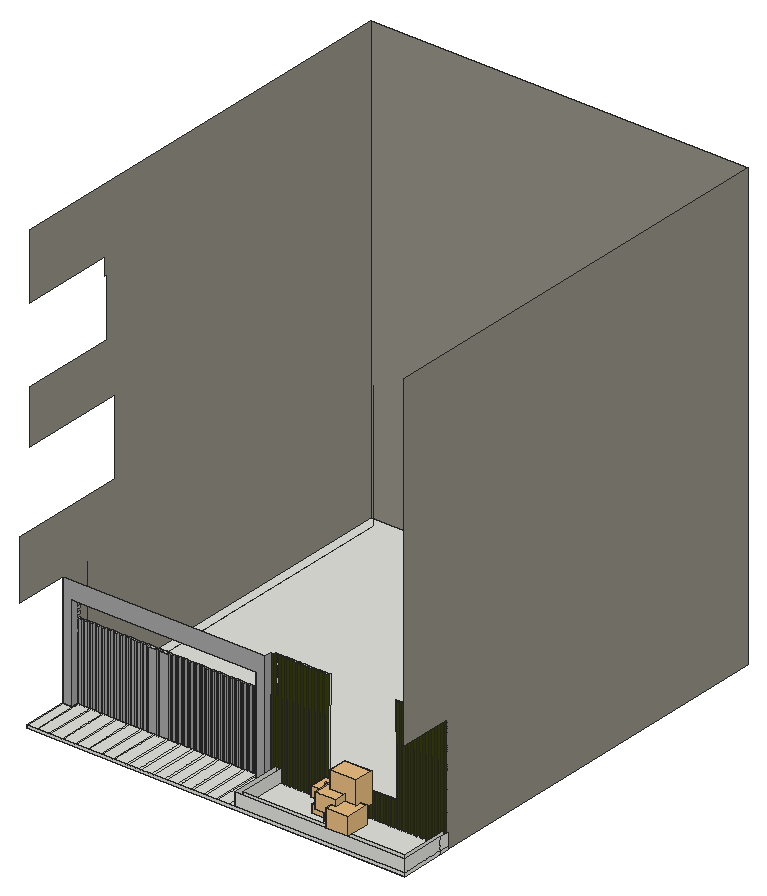
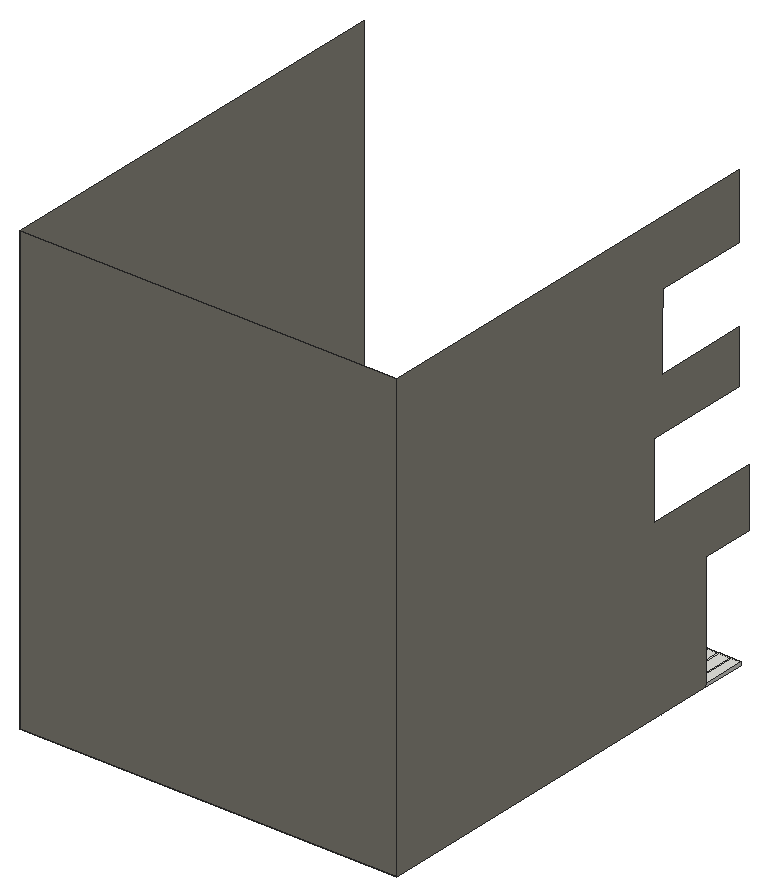
# SketchUp Ruby script. Lengths in inches.
U = 1.inch
M = Sketchup.active_model
def pt(a) = Geom::Point3d.new(a.map { |v| v * U })
def face(e, loops, mat)
  f = e.add_face(loops[0].map { |a| pt(a) })
  loops[1..].each { |l| e.add_face(l.map { |a| pt(a) }).erase! }
  f.material = f.back_material = mat if mat
  f
end
# faces: each face lists its corners as indices into pts; further lists are holes
def faces(e, pts, list, mat = nil) = list.each { |f| face(e, (f[0].is_a?(Array) ? f : [f]).map { |l| l.map { |i| pts[i] } }, mat) }
# xy, xz, yz: faces in a plane at the given z, y or x. An outline is a flat list of corners, or four numbers for a rectangle; further outlines are holes
def ring(l) = l.size == 4 ? [[l[0], l[1]], [l[2], l[1]], [l[2], l[3]], [l[0], l[3]]] : l.each_slice(2).to_a
def flat(e, list, mat, &to3) = list.each { |f| face(e, (f[0].is_a?(Array) ? f : [f]).map { |l| ring(l).map { |u, v| to3.(u, v) } }, mat) }
def xy(e, z, list, mat = nil) = flat(e, list, mat) { |x, y| [x, y, z] }
def xz(e, y, list, mat = nil) = flat(e, list, mat) { |x, z| [x, y, z] }
def yz(e, x, list, mat = nil) = flat(e, list, mat) { |y, z| [x, y, z] }
def lines(e, pts, list) = list.each { |a, b| e.add_line(pt(pts[a]), pt(pts[b])) }
# prism: a flat outline (further loops are holes) pulled along v
def prism(e, loops, v, mat = nil)
  f = face(e, loops, mat); d = Geom::Vector3d.new(v.map { |x| x * U })
  f.pushpull(f.normal.samedirection?(d) ? d.length : -d.length)
end
def box(e, o, s, mat = nil) = prism(e, [[o, [o[0] + s[0], o[1], o[2]], [o[0] + s[0], o[1] + s[1], o[2]], [o[0], o[1] + s[1], o[2]]]], [0, 0, s[2]], mat)
def at(x, y, z, deg = 0) = Geom::Transformation.translation(pt([x, y, z])) * Geom::Transformation.rotation(ORIGIN, Z_AXIS, deg.degrees)
def axes(o, x, y, z) = Geom::Transformation.new([*x, 0, *y, 0, *z, 0, *pt(o).to_a, 1])
def part(name) = M.definitions.add(name)
# library, detail: a bought-in or finely detailed component or shape, given as its bounding box
def library(name, o, s) = part(name).tap { |d| box(d.entities, o, s) }
def detail(e, o, s) = box(e.add_group.entities, o, s)
def put(e, d, t, mat = nil) = e.add_instance(d, t).tap { |i| i.material = mat if mat }
def group(e, t, mat = nil) = e.add_group.tap { |g| g.transformation = t; g.material = mat if mat }.entities
root = M.entities
M.materials.add("Material__1").color = [95, 70, 46]
M.materials.add("Material__2").color = [150, 168, 104]
M.materials.add("Material__3").color = [234, 233, 231]
M.materials.add("Material__4").color = [36, 36, 36]
M.materials.add("Material__5").color = [151, 172, 33]
M.materials.add("Material__6").color = [79, 108, 5]
M.materials.add("[0043_SaddleBrown]1").color = [58, 63, 9]
M.materials.add("[0132_LightGray]").color = [169, 169, 169]
M.materials.add("[Formica Graystone]").color = [149, 146, 135]
M.materials.add("[Polished Concrete Old]").color = [168, 168, 168]
M.materials.add("wire_1").color = [140, 184, 58]
M.materials.add("wire_2").color = [244, 244, 244]
M.materials.add("wire_4").color = [86, 225, 198]
M.materials.add("wire_5").color = [232, 232, 232]
c1 = library("Group\#1",[-915.9375,-34.5,735.6],[41.04,40.85,6.81])
c2 = library("Group\#2",[-991.92,-34.05,729.49],[10.64,7.28,57.53])
c3 = library("Group\#3",[-1022.2,-71.69,736.68],[86.94,78.77,45.64])
c4 = library("Group\#4",[-877.77,-100.41,669.81],[37.9,37.9,42.75])
c5 = library("Group\#5",[-957.79,-83.08,701.98],[44.29,44.29,27.78])
c6 = library("Group\#6",[-1023.9,-65.47,669.625],[67.53,67.55,39.17])
c7 = library("Group\#7",[-997.48,-49.45,708.79],[29.81,29.81,30.61])
c8 = library("Group\#8",[-956738.95,-82059.81,669752.625],[42194.58,42232.57,49521.48])
c9 = library("Group\#9",[-917.52,-36.6875,711.84],[44.99,44.98,28.22])
c10 = library("Group\#10",[-916244.63,-35413.97,669800.48],[42442.38,42642.99,59706.29])
c11 = library("Group\#11",[-955.48,-54.29,730.4],[118.63,83.7,130.4])
c12 = library("Group\#12",[-899.97,-18.72,732.17],[8.78,8.27,28.64])
c13 = library("Group\#13",[-906.16,-138.28,686.8],[98.25,106.18,75.79])
c14 = library("Group\#14",[-978.71,-103.24,719.12],[90.2,76.4,68.29])
c15 = library("Group\#15",[-955.98,-81.17,725.57],[41.03,40.85,6.81])
c16 = library("Group\#16",[-996.8,-48.73,736.67],[28.51,28.38,4.73])
c17 = library("Group\#17",[-876.58,-99.29,706.19],[35.74,35.58,5.93])
c18 = library("Group\#18",[-912.1,-32.49,735.82],[33.14,36.63,9.55])
c19 = library("Group\#19",[-994.36,-46.95,735.88],[24.38,25.9,6.88])
c20 = part("PLANT-30")
p = [[0,0,0],[1,0,0],[1,1,0]]
lines(c20.entities,p,[[0,1],[1,2],[2,0]])
put(c20.entities,c1,at(895.63,-7.06,-669.82),"Material__1")
put(c20.entities,c2,at(895.63,-7.06,-669.82),"wire_1")
put(c20.entities,c3,at(895.63,-7.06,-669.82),"Material__2")
put(c20.entities,c4,at(895.63,-7.06,-669.82),"wire_2")
put(c20.entities,c5,at(895.63,-7.06,-669.82),"wire_2")
put(c20.entities,c6,at(895.63,-7.06,-669.82),"Material__3")
put(c20.entities,c7,at(895.63,-7.06,-669.82),"wire_2")
put(c20.entities,c8,axes([895.63,-7.06,-669.82],[0.001,0,0],[0,0.001,0],[0,0,0.001]),"Material__4")
put(c20.entities,c9,at(895.63,-7.06,-669.82),"wire_2")
put(c20.entities,c10,axes([895.63,-7.06,-669.82],[0.001,0,0],[0,0.001,0],[0,0,0.001]),"Material__4")
put(c20.entities,c11,at(895.63,-7.06,-669.82),"Material__5")
put(c20.entities,c12,at(895.63,-7.06,-669.82),"wire_4")
put(c20.entities,c13,at(895.63,-7.06,-669.82),"Material__6")
put(c20.entities,c14,at(895.63,-7.06,-669.82),"Material__4")
put(c20.entities,c15,at(895.63,-7.06,-669.82),"Material__1")
put(c20.entities,c16,at(895.63,-7.06,-669.82),"Material__1")
put(c20.entities,c17,at(895.63,-7.06,-669.82),"Material__1")
put(c20.entities,c18,at(895.63,-7.06,-669.82),"wire_5")
put(c20.entities,c19,at(895.63,-7.06,-669.82),"wire_5")
xy(root,0,[[0,17.5625,361.1875,60],[0,60,0,429,360,429,360,69,196.36,69,196.36,68.9375,193.125,68.9375,193.125,69,8.86,69,8.86,60],[8.86,60,184.43,66],[184.43,60,193.125,69],[193.125,60,193.125,67,196.36,67,196.36,68.9375,198.375,68.9375,198.375,67,201.61,67,201.61,68.9375,203.625,68.9375,203.625,67,206.86,67,206.86,68.9375,208.875,68.9375,208.875,67,212.11,67,212.11,68.9375,214.125,68.9375,214.125,67,217.36,67,217.36,68.9375,219.375,68.9375,219.375,67,222.61,67,222.61,68.9375,224.625,68.9375,224.625,67,227.86,67,227.86,68.9375,229.875,68.9375,229.875,67,233.11,67,233.11,68.9375,235.125,68.9375,235.125,67,238.36,67,238.36,68.9375,240.375,68.9375,240.375,67,243.61,67,243.61,68.9375,245.625,68.9375,245.625,67,248.86,67,248.86,68.9375,250.875,68.9375,250.875,67,254.11,67,254.11,68.9375,256.125,68.9375,256.125,67,259.36,67,259.36,68.9375,261.375,68.9375,261.375,67,264.61,67,264.61,68.9375,266.625,68.9375,266.625,67,269.86,67,269.86,68.9375,271.875,68.9375,271.875,67,275.11,67,275.11,68.9375,277.125,68.9375,277.125,67,280.36,67,280.36,68.9375,282.375,68.9375,282.375,67,285.61,67,285.61,68.9375,287.625,68.9375,287.625,67,290.86,67,290.86,68.9375,292.875,68.9375,292.875,67,296.11,67,296.11,68.9375,298.125,68.9375,298.125,67,301.36,67,301.36,68.9375,303.375,68.9375,303.375,67,306.61,67,306.61,68.9375,308.625,68.9375,308.625,67,311.86,67,311.86,68.9375,313.875,68.9375,313.875,67,317.11,67,317.11,68.9375,319.125,68.9375,319.125,67,322.36,67,322.36,68.9375,324.375,68.9375,324.375,67,327.61,67,327.61,68.9375,330.125,68.9375,330.125,67,333.36,67,333.36,68.9375,335.875,68.9375,335.875,67,339.11,67,339.11,68.9375,341.625,68.9375,341.625,67,344.86,67,344.86,68.9375,347.375,68.9375,347.375,67,350.61,67,350.61,68.9375,353.125,68.9375,353.125,67,356.36,67,356.36,68.9375,358.875,68.9375,358.875,67,360,67,360,68.9375,361.1875,68.9375,361.1875,60],
  [76.57,66,85.45,69],[87.63,66,96.52,69],[8.86,67,12.35,69],[14.55,67,18.04,69],[20.24,67,23.72,69],
  [25.93,67,29.41,69],[31.61,67,35.1,69],[37.3,67,40.79,69],[42.99,67,46.47,69],[48.68,67,52.16,69],
  [54.36,67,57.85,69],[60.05,67,63.54,69],[65.74,67,69.22,69],[71.43,67,74.91,69],[97.66,67,99.86,69],
  [103.35,67,105.55,69],[109.04,67,111.24,69],[114.72,67,116.93,69],[120.41,67,122.61,69],[126.1,67,128.3,69],
  [131.79,67,133.99,69],[137.47,67,139.68,69],[143.16,67,145.36,69],[148.85,67,151.05,69],[154.54,67,156.74,69],
  [160.22,67,162.43,69],[165.91,67,168.11,69],[171.6,67,173.8,69],[177.29,67,179.49,69],[182.97,67,184.43,69],
  [193.125,67,196.36,68.9375],[198.375,67,201.61,68.9375],[203.625,67,206.86,68.9375],[208.875,67,212.11,68.9375],[214.125,67,217.36,68.9375],
  [219.375,67,222.61,68.9375],[224.625,67,227.86,68.9375],[229.875,67,233.11,68.9375],[235.125,67,238.36,68.9375],[240.375,67,243.61,68.9375],
  [245.625,67,248.86,68.9375],[250.875,67,254.11,68.9375],[256.125,67,259.36,68.9375],[261.375,67,264.61,68.9375],[266.625,67,269.86,68.9375],
  [271.875,67,275.11,68.9375],[277.125,67,280.36,68.9375],[282.375,67,285.61,68.9375],[287.625,67,290.86,68.9375],[292.875,67,296.11,68.9375],
  [298.125,67,301.36,68.9375],[303.375,67,306.61,68.9375],[308.625,67,311.86,68.9375],[313.875,67,317.11,68.9375],[319.125,67,322.36,68.9375],
  [324.375,67,327.61,68.9375],[330.125,67,333.36,68.9375],[335.875,67,339.11,68.9375],[341.625,67,344.86,68.9375],[347.375,67,350.61,68.9375],
  [353.125,67,356.36,68.9375],[358.875,67,360,68.9375],[198.375,68.9375,201.61,69],[203.625,68.9375,206.86,69],[208.875,68.9375,212.11,69],
  [214.125,68.9375,217.36,69],[219.375,68.9375,222.61,69],[224.625,68.9375,227.86,69],[229.875,68.9375,233.11,69],[235.125,68.9375,238.36,69],
  [240.375,68.9375,243.61,69],[245.625,68.9375,248.86,69],[250.875,68.9375,254.11,69],[256.125,68.9375,259.36,69],[261.375,68.9375,264.61,69],
  [266.625,68.9375,269.86,69],[271.875,68.9375,275.11,69],[277.125,68.9375,280.36,69],[282.375,68.9375,285.61,69],[287.625,68.9375,290.86,69],
  [292.875,68.9375,296.11,69],[298.125,68.9375,301.36,69],[303.375,68.9375,306.61,69],[308.625,68.9375,311.86,69],[313.875,68.9375,317.11,69],
  [319.125,68.9375,322.36,69],[324.375,68.9375,327.61,69],[330.125,68.9375,333.36,69],[335.875,68.9375,339.11,69],[341.625,68.9375,344.86,69],
  [347.375,68.9375,350.61,69],[353.125,68.9375,356.36,69],[358.875,68.9375,360,69]])
xy(root,3,[[0,17.5625,9.02,60],[9.02,17.5625,10.37,17.5625,10.37,66,8.86,66,8.86,60,9.02,60],[10.37,17.5625,20.81,66],[20.81,17.5625,22.68,66],[22.68,17.5625,33.12,66],
  [33.12,17.5625,35,66],[35,17.5625,45.43,66],[45.43,17.5625,47.31,66],[47.31,17.5625,57.75,66],[57.75,17.5625,59.62,66],
  [59.62,17.5625,70.06,66],[70.06,17.5625,71.93,66],[71.93,17.5625,82.37,66],[82.37,17.5625,84.25,66],[84.25,17.5625,94.68,66],
  [94.68,17.5625,96.56,66],[96.56,17.5625,107,66],[107,17.5625,108.87,66],[108.87,17.5625,119.31,66],[119.31,17.5625,121.18,66],
  [121.18,17.5625,131.62,66],[131.62,17.5625,133.5,66],[133.5,17.5625,143.93,66],[143.93,17.5625,145.81,66],[145.81,17.5625,156.25,66],
  [156.25,17.5625,158.12,66],[158.12,17.5625,168.56,66],[168.56,17.5625,170.43,66],[170.43,17.5625,180.87,66],[180.87,17.5625,182.75,66],
  [182.75,17.5625,193.18,17.5625,193.18,66,193.125,66,193.125,60,184.43,60,184.43,66,182.75,66],[193.18,17.5625,198.375,17.5625,198.375,67,202.875,67,202.875,22.19,357.51,22.19,357.51,68.9375,193.125,68.9375,193.125,66,193.18,66],[198.375,17.5625,198.375,67,202.875,67,202.875,22.19,357.51,22.19,357.51,68.9375,361.1875,68.9375,361.1875,17.5625],[184.43,60,193.125,66]])
xz(root,17.5625,[[0,0,361.1875,3],[198.375,3,361.1875,15]])
xz(root,22.19,[[202.875,3,357.51,15]])
xz(root,60,[[0,0,8.86,3],[184.43,0,193.125,3]])
xz(root,60,[[0,3,8.86,3,8.86,94.26,184.43,94.26,184.43,3,193.125,3,193.125,111.13,0,111.13]],"[Polished Concrete Old]")
xz(root,66,[[8.86,0,76.57,3],[76.57,0,85.45,3],[85.45,0,87.63,3],[87.63,0,96.52,3],[96.52,0,184.43,3]])
xz(root,66,[[76.57,3,85.45,3,85.45,51.4,85.07,51.4,85.07,52.46,85.45,52.46,85.45,57.65,85.07,57.65,85.07,58.71,85.45,58.71,85.45,75.79,76.57,75.79],[87.63,3,96.52,3,96.52,75.79,87.63,75.79,87.63,58.71,88.01,58.71,88.01,57.65,87.63,57.65,87.63,52.46,88.01,52.46,88.01,51.4,87.63,51.4]],"[0132_LightGray]")
xz(root,67,[[198.375,0,201.61,3],[198.375,3,201.61,15],[201.61,3,202.875,15]])
xz(root,67,[[193.125,0,196.36,111.13],[203.625,0,206.86,111.13],[208.875,0,212.11,111.13],[214.125,0,217.36,111.13],[219.375,0,222.61,111.13],
  [224.625,0,227.86,111.13],[229.875,0,233.11,111.13],[235.125,0,238.36,111.13],[240.375,0,243.61,111.13],[245.625,0,248.86,0,248.86,26.18,248.25,26.18,248.25,84.93,248.86,84.93,248.86,111.13,245.625,111.13],
  [250.875,0,254.11,26.18],[256.125,0,259.36,26.18],[261.375,0,264.61,26.18],[266.625,0,269.86,26.18],[271.875,0,275.11,26.18],
  [277.125,0,280.36,26.18],[282.375,0,285.61,26.18],[287.625,0,290.86,26.18],[292.875,0,296.11,26.18],[298.125,0,301.36,26.18],
  [303.375,0,306.61,26.18],[308.625,0,311.86,26.18],[313.875,0,317.11,111.13],[319.125,0,322.36,111.13],[324.375,0,327.61,111.13],
  [330.125,0,333.36,111.13],[335.875,0,339.11,111.13],[341.625,0,344.86,111.13],[347.375,0,350.61,111.13],[353.125,0,356.36,111.13],
  [358.875,0,360,111.13]],"[0043_SaddleBrown]1")
xz(root,67,[[8.86,0,12.35,75.79],[14.55,0,18.04,75.79],[20.24,0,23.72,75.79],[25.93,0,29.41,75.79],[31.61,0,35.1,75.79],
  [37.3,0,40.79,75.79],[42.99,0,46.47,75.79],[48.68,0,52.16,75.79],[54.36,0,57.85,75.79],[60.05,0,63.54,75.79],
  [65.74,0,69.22,75.79],[71.43,0,74.91,75.79],[97.66,0,99.86,75.79],[103.35,0,105.55,75.79],[109.04,0,111.24,75.79],
  [114.72,0,116.93,75.79],[120.41,0,122.61,75.79],[126.1,0,128.3,75.79],[131.79,0,133.99,75.79],[137.47,0,139.68,75.79],
  [143.16,0,145.36,75.79],[148.85,0,151.05,75.79],[154.54,0,156.74,75.79],[160.22,0,162.43,75.79],[165.91,0,168.11,75.79],
  [171.6,0,173.8,75.79],[177.29,0,179.49,75.79],[182.97,0,184.43,75.79]],"[0132_LightGray]")
xz(root,68.9375,[[193.125,0,361.1875,3],[357.51,3,361.1875,15]])
xz(root,69,[[8.86,0,12.35,75.79],[14.55,0,18.04,75.79],[20.24,0,23.72,75.79],[25.93,0,29.41,75.79],[31.61,0,35.1,75.79],
  [37.3,0,40.79,75.79],[42.99,0,46.47,75.79],[48.68,0,52.16,75.79],[54.36,0,57.85,75.79],[60.05,0,63.54,75.79],
  [65.74,0,69.22,75.79],[71.43,0,74.91,75.79],[76.57,0,77.11,75.79],[77.11,0,80.6,75.79],[80.6,0,82.8,75.79],
  [82.8,0,85.45,75.79],[87.63,0,88.49,75.79],[88.49,0,91.97,75.79],[91.97,0,94.18,75.79],[94.18,0,96.52,75.79],
  [97.66,0,99.86,75.79],[103.35,0,105.55,75.79],[109.04,0,111.24,75.79],[114.72,0,116.93,75.79],[120.41,0,122.61,75.79],
  [126.1,0,128.3,75.79],[131.79,0,133.99,75.79],[137.47,0,139.68,75.79],[143.16,0,145.36,75.79],[148.85,0,151.05,75.79],
  [154.54,0,156.74,75.79],[160.22,0,162.43,75.79],[165.91,0,168.11,75.79],[171.6,0,173.8,75.79],[177.29,0,179.49,75.79],
  [182.97,0,184.43,75.79],[185.18,0,188.66,75.79],[190.86,0,193.125,75.79],[196.36,0,198.375,111.13],[198.375,0,201.61,111.13],
  [201.61,0,203.625,111.13],[203.625,0,206.86,111.13],[206.86,0,208.875,111.13],[208.875,0,212.11,111.13],[212.11,0,214.125,111.13],
  [214.125,0,217.36,111.13],[217.36,0,219.375,111.13],[219.375,0,222.61,111.13],[222.61,0,224.625,111.13],[224.625,0,227.86,111.13],
  [227.86,0,229.875,111.13],[229.875,0,233.11,111.13],[233.11,0,235.125,111.13],[235.125,0,238.36,111.13],[238.36,0,240.375,111.13],
  [240.375,0,243.61,111.13],[243.61,0,245.625,111.13],[245.625,0,245.625,111.13,248.86,111.13,248.86,84.93,248.25,84.93,248.25,26.18,248.86,26.18,248.86,0],[248.86,0,250.875,26.18],[250.875,0,254.11,26.18],
  [254.11,0,256.125,26.18],[256.125,0,259.36,26.18],[259.36,0,261.375,26.18],[261.375,0,264.61,26.18],[264.61,0,266.625,26.18],
  [266.625,0,269.86,26.18],[269.86,0,271.875,26.18],[271.875,0,275.11,26.18],[275.11,0,277.125,26.18],[277.125,0,280.36,26.18],
  [280.36,0,282.375,26.18],[282.375,0,285.61,26.18],[285.61,0,287.625,26.18],[287.625,0,290.86,26.18],[290.86,0,292.875,26.18],
  [292.875,0,296.11,26.18],[296.11,0,298.125,26.18],[298.125,0,301.36,26.18],[301.36,0,303.375,26.18],[303.375,0,306.61,26.18],
  [306.61,0,308.625,26.18],[308.625,0,311.86,26.18],[311.86,0,313.875,0,313.875,111.13,311.86,111.13,311.86,84.93,312.4375,84.93,312.4375,26.18,311.86,26.18],[313.875,0,317.11,111.13],[317.11,0,319.125,111.13],
  [319.125,0,322.36,111.13],[322.36,0,324.375,111.13],[324.375,0,327.61,111.13],[327.61,0,330.125,111.13],[330.125,0,333.36,111.13],
  [333.36,0,335.875,111.13],[335.875,0,339.11,111.13],[339.11,0,341.625,111.13],[341.625,0,344.86,111.13],[344.86,0,347.375,111.13],
  [347.375,0,350.61,111.13],[350.61,0,353.125,111.13],[353.125,0,356.36,111.13],[358.875,0,360,111.13]])
xz(root,69,[[356.36,0,358.875,111.13]],"[0043_SaddleBrown]1")
xz(root,69,[[12.35,0,14.55,75.79],[18.04,0,20.24,75.79],[23.72,0,25.93,75.79],[29.41,0,31.61,75.79],[35.1,0,37.3,75.79],
  [40.79,0,42.99,75.79],[46.47,0,48.68,75.79],[52.16,0,54.36,75.79],[57.85,0,60.05,75.79],[63.54,0,65.74,75.79],
  [69.22,0,71.43,75.79],[74.91,0,76.57,75.79],[85.45,0,86.29,75.79],[86.29,0,87.63,75.79],[96.52,0,97.66,75.79],
  [99.86,0,103.35,75.79],[105.55,0,109.04,75.79],[111.24,0,114.72,75.79],[116.93,0,120.41,75.79],[122.61,0,126.1,75.79],
  [128.3,0,131.79,75.79],[133.99,0,137.47,75.79],[139.68,0,143.16,75.79],[145.36,0,148.85,75.79],[151.05,0,154.54,75.79],
  [156.74,0,160.22,75.79],[162.43,0,165.91,75.79],[168.11,0,171.6,75.79],[173.8,0,177.29,75.79],[179.49,0,182.97,75.79]],"[0132_LightGray]")
xz(root,265.8125,[[219.375,0,222.61,111.13]])
xz(root,429,[[0,0,360,426]],"[Formica Graystone]")
yz(root,0,[[17.5625,0,60,3]])
yz(root,0,[[60,0,60,111.13,9,111.13,9,168,21,168,21,168.11,121.875,168.11,121.875,240,21,240,21,291,112.875,291,112.875,346.66,110.875,346.66,110.875,363,21,363,21,426,429,426,429,0]],"[Formica Graystone]")
yz(root,8.86,[[60,0,66,3],[67,0,69,75.79]])
yz(root,8.86,[[66,0,67,0,67,75.79,66,75.79,66,78.7,69,78.7,69,80.98,66,80.98,66,83.88,69,83.88,69,86.17,66,86.17,66,89.07,69,89.07,69,91.35,66,91.35,66,94.26,60,94.26,60,3,66,3]],"[Polished Concrete Old]")
yz(root,12.35,[[67,0,69,75.79]],"[0132_LightGray]")
yz(root,14.55,[[67,0,69,75.79]],"[0132_LightGray]")
yz(root,18.04,[[67,0,69,75.79]],"[0132_LightGray]")
yz(root,20.24,[[67,0,69,75.79]],"[0132_LightGray]")
yz(root,23.72,[[67,0,69,75.79]],"[0132_LightGray]")
yz(root,25.93,[[67,0,69,75.79]],"[0132_LightGray]")
yz(root,29.41,[[67,0,69,75.79]],"[0132_LightGray]")
yz(root,31.61,[[67,0,69,75.79]],"[0132_LightGray]")
yz(root,35.1,[[67,0,69,75.79]],"[0132_LightGray]")
yz(root,37.3,[[67,0,69,75.79]],"[0132_LightGray]")
yz(root,40.79,[[67,0,69,75.79]],"[0132_LightGray]")
yz(root,42.99,[[67,0,69,75.79]],"[0132_LightGray]")
yz(root,46.47,[[67,0,69,75.79]],"[0132_LightGray]")
yz(root,48.68,[[67,0,69,75.79]],"[0132_LightGray]")
yz(root,52.16,[[67,0,69,75.79]],"[0132_LightGray]")
yz(root,54.36,[[67,0,69,75.79]],"[0132_LightGray]")
yz(root,57.85,[[67,0,69,75.79]],"[0132_LightGray]")
yz(root,60.05,[[67,0,69,75.79]],"[0132_LightGray]")
yz(root,63.54,[[67,0,69,75.79]],"[0132_LightGray]")
yz(root,65.74,[[67,0,69,75.79]],"[0132_LightGray]")
yz(root,69.22,[[67,0,69,75.79]],"[0132_LightGray]")
yz(root,71.43,[[67,0,69,75.79]],"[0132_LightGray]")
yz(root,74.91,[[67,0,69,75.79]],"[0132_LightGray]")
yz(root,76.57,[[66,0,69,75.79]],"[0132_LightGray]")
yz(root,85.45,[[66,0,69,75.79]],"[0132_LightGray]")
yz(root,87.63,[[66,0,69,75.79]],"[0132_LightGray]")
yz(root,96.52,[[66,0,69,75.79]],"[0132_LightGray]")
yz(root,97.66,[[67,0,69,75.79]],"[0132_LightGray]")
yz(root,99.86,[[67,0,69,75.79]],"[0132_LightGray]")
yz(root,103.35,[[67,0,69,75.79]],"[0132_LightGray]")
yz(root,105.55,[[67,0,69,75.79]],"[0132_LightGray]")
yz(root,109.04,[[67,0,69,75.79]],"[0132_LightGray]")
yz(root,111.24,[[67,0,69,75.79]],"[0132_LightGray]")
yz(root,114.72,[[67,0,69,75.79]],"[0132_LightGray]")
yz(root,116.93,[[67,0,69,75.79]],"[0132_LightGray]")
yz(root,120.41,[[67,0,69,75.79]],"[0132_LightGray]")
yz(root,122.61,[[67,0,69,75.79]],"[0132_LightGray]")
yz(root,126.1,[[67,0,69,75.79]],"[0132_LightGray]")
yz(root,128.3,[[67,0,69,75.79]],"[0132_LightGray]")
yz(root,131.79,[[67,0,69,75.79]],"[0132_LightGray]")
yz(root,133.99,[[67,0,69,75.79]],"[0132_LightGray]")
yz(root,137.47,[[67,0,69,75.79]],"[0132_LightGray]")
yz(root,139.68,[[67,0,69,75.79]],"[0132_LightGray]")
yz(root,143.16,[[67,0,69,75.79]],"[0132_LightGray]")
yz(root,145.36,[[67,0,69,75.79]],"[0132_LightGray]")
yz(root,148.85,[[67,0,69,75.79]],"[0132_LightGray]")
yz(root,151.05,[[67,0,69,75.79]],"[0132_LightGray]")
yz(root,154.54,[[67,0,69,75.79]],"[0132_LightGray]")
yz(root,156.74,[[67,0,69,75.79]],"[0132_LightGray]")
yz(root,160.22,[[67,0,69,75.79]],"[0132_LightGray]")
yz(root,162.43,[[67,0,69,75.79]],"[0132_LightGray]")
yz(root,165.91,[[67,0,69,75.79]],"[0132_LightGray]")
yz(root,168.11,[[67,0,69,75.79]],"[0132_LightGray]")
yz(root,171.6,[[67,0,69,75.79]],"[0132_LightGray]")
yz(root,173.8,[[67,0,69,75.79]],"[0132_LightGray]")
yz(root,177.29,[[67,0,69,75.79]],"[0132_LightGray]")
yz(root,179.49,[[67,0,69,75.79]],"[0132_LightGray]")
yz(root,182.97,[[67,0,69,75.79]],"[0132_LightGray]")
yz(root,184.43,[[60,0,66,3],[67,0,69,75.79]])
yz(root,184.43,[[66,0,66,3,60,3,60,94.26,66,94.26,66,91.35,69,91.35,69,89.07,66,89.07,66,86.17,69,86.17,69,83.88,66,83.88,66,80.98,69,80.98,69,78.7,66,78.7,66,75.79,67,75.79,67,0]],"[Polished Concrete Old]")
yz(root,193.125,[[60,0,67,3],[67,0,68.9375,3],[68.9375,0,69,0,69,75.79,67,75.79,67,3,68.9375,3]])
yz(root,193.125,[[60,3,67,111.13]],"[Polished Concrete Old]")
yz(root,196.36,[[67,0,69,111.13]],"[0043_SaddleBrown]1")
yz(root,198.375,[[17.5625,3,67,15]])
yz(root,198.375,[[67,0,69,75.79]],"[0043_SaddleBrown]1")
yz(root,201.61,[[67,0,69,111.13]],"[0043_SaddleBrown]1")
yz(root,202.875,[[22.19,3,67,15]])
yz(root,203.625,[[67,0,69,75.79]],"[0043_SaddleBrown]1")
yz(root,206.86,[[67,0,69,111.13]],"[0043_SaddleBrown]1")
yz(root,208.875,[[67,0,69,75.79]],"[0043_SaddleBrown]1")
yz(root,212.11,[[67,0,69,111.13]],"[0043_SaddleBrown]1")
yz(root,214.125,[[67,0,69,75.79]],"[0043_SaddleBrown]1")
yz(root,217.36,[[67,0,69,111.13]],"[0043_SaddleBrown]1")
yz(root,219.375,[[67,0,69,75.79]],"[0043_SaddleBrown]1")
yz(root,222.61,[[67,0,69,111.13]],"[0043_SaddleBrown]1")
yz(root,224.625,[[67,0,69,75.79]],"[0043_SaddleBrown]1")
yz(root,227.86,[[67,0,69,111.13]],"[0043_SaddleBrown]1")
yz(root,229.875,[[67,0,69,75.79]],"[0043_SaddleBrown]1")
yz(root,233.11,[[67,0,69,111.13]],"[0043_SaddleBrown]1")
yz(root,235.125,[[67,0,69,75.79]],"[0043_SaddleBrown]1")
yz(root,238.36,[[67,0,69,111.13]],"[0043_SaddleBrown]1")
yz(root,240.375,[[67,0,69,75.79]],"[0043_SaddleBrown]1")
yz(root,243.61,[[67,0,69,111.13]],"[0043_SaddleBrown]1")
yz(root,245.625,[[67,0,69,75.79]],"[0043_SaddleBrown]1")
yz(root,248.86,[[67,0,69,26.18]],"[0043_SaddleBrown]1")
yz(root,250.875,[[67,0,69,26.18]],"[0043_SaddleBrown]1")
yz(root,254.11,[[67,0,69,26.18]],"[0043_SaddleBrown]1")
yz(root,256.125,[[67,0,69,26.18]],"[0043_SaddleBrown]1")
yz(root,259.36,[[67,0,69,26.18]],"[0043_SaddleBrown]1")
yz(root,261.375,[[67,0,69,26.18]],"[0043_SaddleBrown]1")
yz(root,264.61,[[67,0,69,26.18]],"[0043_SaddleBrown]1")
yz(root,266.625,[[67,0,69,26.18]],"[0043_SaddleBrown]1")
yz(root,269.86,[[67,0,69,26.18]])
yz(root,271.875,[[67,0,69,26.18]],"[0043_SaddleBrown]1")
yz(root,275.11,[[67,0,69,26.18]])
yz(root,277.125,[[67,0,69,26.18]],"[0043_SaddleBrown]1")
yz(root,280.36,[[67,0,69,26.18]],"[0043_SaddleBrown]1")
yz(root,282.375,[[67,0,69,26.18]],"[0043_SaddleBrown]1")
yz(root,285.61,[[67,0,69,26.18]],"[0043_SaddleBrown]1")
yz(root,287.625,[[67,0,69,26.18]],"[0043_SaddleBrown]1")
yz(root,290.86,[[67,0,69,26.18]],"[0043_SaddleBrown]1")
yz(root,292.875,[[67,0,69,26.18]],"[0043_SaddleBrown]1")
yz(root,296.11,[[67,0,69,26.18]],"[0043_SaddleBrown]1")
yz(root,298.125,[[67,0,69,26.18]],"[0043_SaddleBrown]1")
yz(root,301.36,[[67,0,69,26.18]],"[0043_SaddleBrown]1")
yz(root,303.375,[[67,0,69,26.18]],"[0043_SaddleBrown]1")
yz(root,306.61,[[67,0,69,26.18]],"[0043_SaddleBrown]1")
yz(root,308.625,[[67,0,69,26.18]],"[0043_SaddleBrown]1")
yz(root,311.86,[[67,0,69,26.18]],"[0043_SaddleBrown]1")
yz(root,313.875,[[67,0,69,75.79]],"[0043_SaddleBrown]1")
yz(root,317.11,[[67,0,69,111.13]],"[0043_SaddleBrown]1")
yz(root,319.125,[[67,0,69,75.79]],"[0043_SaddleBrown]1")
yz(root,322.36,[[67,0,69,111.13]],"[0043_SaddleBrown]1")
yz(root,324.375,[[67,0,69,75.79]],"[0043_SaddleBrown]1")
yz(root,327.61,[[67,0,69,111.13]],"[0043_SaddleBrown]1")
yz(root,330.125,[[67,0,69,75.79]],"[0043_SaddleBrown]1")
yz(root,333.36,[[67,0,69,111.13]],"[0043_SaddleBrown]1")
yz(root,335.875,[[67,0,69,75.79]],"[0043_SaddleBrown]1")
yz(root,339.11,[[67,0,69,111.13]],"[0043_SaddleBrown]1")
yz(root,341.625,[[67,0,69,75.79]],"[0043_SaddleBrown]1")
yz(root,344.86,[[67,0,69,111.13]],"[0043_SaddleBrown]1")
yz(root,347.375,[[67,0,69,75.79]],"[0043_SaddleBrown]1")
yz(root,350.61,[[67,0,69,111.13]],"[0043_SaddleBrown]1")
yz(root,351,[[78,0,78,120,195.3125,120,195.3125,240,207,240,207,120,420,120,420,0]])
yz(root,353.125,[[67,0,69,75.79]],"[0043_SaddleBrown]1")
yz(root,356.36,[[67,0,69,111.13]],"[0043_SaddleBrown]1")
yz(root,357.51,[[22.19,3,68.9375,15]])
yz(root,358.875,[[67,0,69,75.79]],"[0043_SaddleBrown]1")
yz(root,360,[[67,0,69,111.13]],"[0043_SaddleBrown]1")
yz(root,360,[[69,0,429,0,429,426,18,426,18,111.13,69,111.13]],"[Formica Graystone]")
yz(root,361.1875,[[17.5625,0,60,3],[60,0,68.9375,3],[17.5625,3,60,15],[60,3,68.9375,15]])
p = [[9,420,0],[9,78,0],[9,420,120],[9,78,120],[0,112.875,0],[0,112.875,-0.78],
  [351,78,0]]
lines(root,p,[[0,1],[0,2],[1,3],[4,5],[1,6]])
put(root,c20,axes([287.54,49.04,11.56],[0.2166,0,0],[0,0.2166,0],[0,0,0.2166]),"[0043_SaddleBrown]1")
